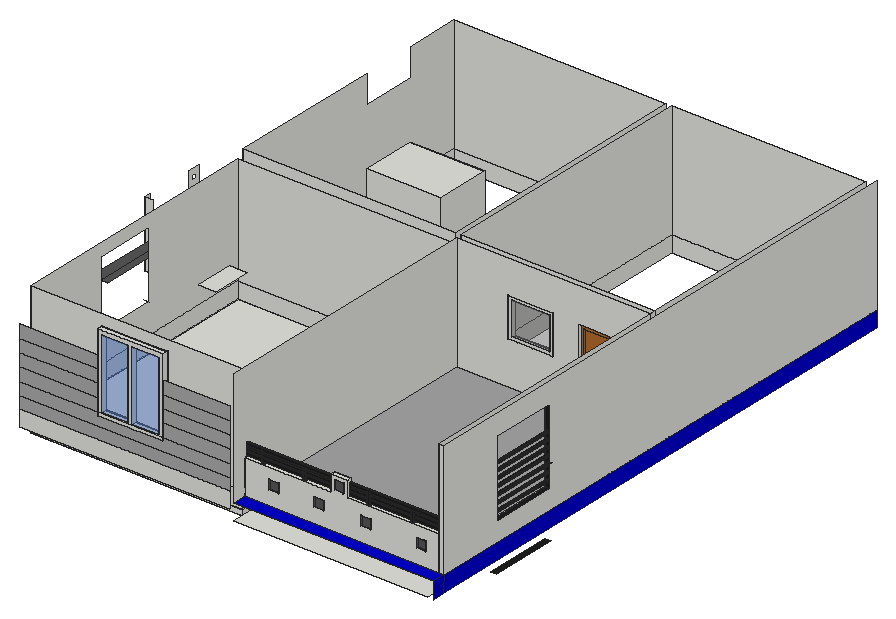
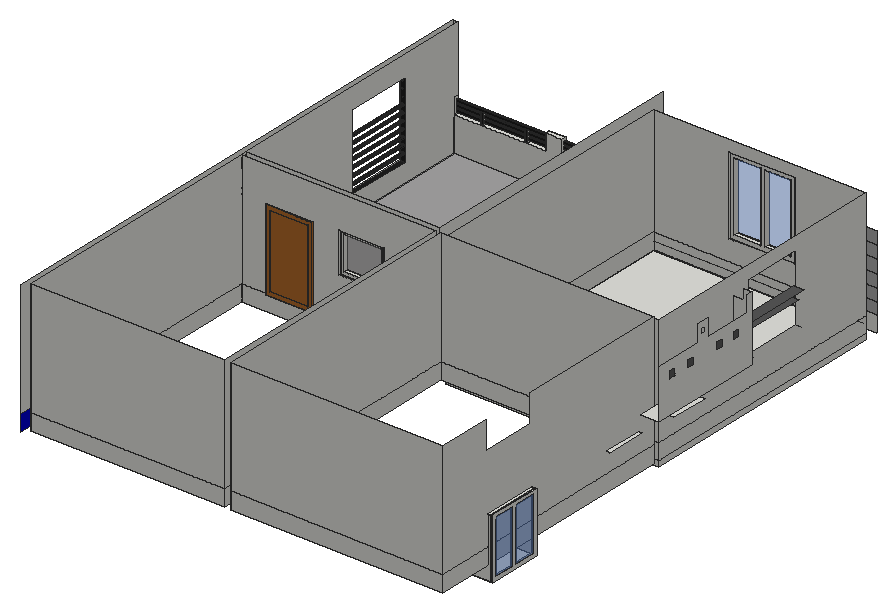
# SketchUp Ruby script. Lengths in inches.
U = 1.inch
M = Sketchup.active_model
def pt(a) = Geom::Point3d.new(a.map { |v| v * U })
def face(e, loops, mat)
  f = e.add_face(loops[0].map { |a| pt(a) })
  loops[1..].each { |l| e.add_face(l.map { |a| pt(a) }).erase! }
  f.material = f.back_material = mat if mat
  f
end
# faces: each face lists its corners as indices into pts; further lists are holes
def faces(e, pts, list, mat = nil) = list.each { |f| face(e, (f[0].is_a?(Array) ? f : [f]).map { |l| l.map { |i| pts[i] } }, mat) }
# xy, xz, yz: faces in a plane at the given z, y or x. An outline is a flat list of corners, or four numbers for a rectangle; further outlines are holes
def ring(l) = l.size == 4 ? [[l[0], l[1]], [l[2], l[1]], [l[2], l[3]], [l[0], l[3]]] : l.each_slice(2).to_a
def flat(e, list, mat, &to3) = list.each { |f| face(e, (f[0].is_a?(Array) ? f : [f]).map { |l| ring(l).map { |u, v| to3.(u, v) } }, mat) }
def xy(e, z, list, mat = nil) = flat(e, list, mat) { |x, y| [x, y, z] }
def xz(e, y, list, mat = nil) = flat(e, list, mat) { |x, z| [x, y, z] }
def yz(e, x, list, mat = nil) = flat(e, list, mat) { |y, z| [x, y, z] }
def lines(e, pts, list) = list.each { |a, b| e.add_line(pt(pts[a]), pt(pts[b])) }
# prism: a flat outline (further loops are holes) pulled along v
def prism(e, loops, v, mat = nil)
  f = face(e, loops, mat); d = Geom::Vector3d.new(v.map { |x| x * U })
  f.pushpull(f.normal.samedirection?(d) ? d.length : -d.length)
end
def box(e, o, s, mat = nil) = prism(e, [[o, [o[0] + s[0], o[1], o[2]], [o[0] + s[0], o[1] + s[1], o[2]], [o[0], o[1] + s[1], o[2]]]], [0, 0, s[2]], mat)
def at(x, y, z, deg = 0) = Geom::Transformation.translation(pt([x, y, z])) * Geom::Transformation.rotation(ORIGIN, Z_AXIS, deg.degrees)
def axes(o, x, y, z) = Geom::Transformation.new([*x, 0, *y, 0, *z, 0, *pt(o).to_a, 1])
def part(name) = M.definitions.add(name)
# library, detail: a bought-in or finely detailed component or shape, given as its bounding box
def library(name, o, s) = part(name).tap { |d| box(d.entities, o, s) }
def detail(e, o, s) = box(e.add_group.entities, o, s)
def put(e, d, t, mat = nil) = e.add_instance(d, t).tap { |i| i.material = mat if mat }
def group(e, t, mat = nil) = e.add_group.tap { |g| g.transformation = t; g.material = mat if mat }.entities
root = M.entities
M.materials.add("[Color I06]").color = [0, 0, 204]
M.materials.add("[Color M03]").color = [170, 170, 170]
M.materials.add("[Color M06]").color = [86, 86, 86]
M.materials.add("[Color M08]").color = [30, 30, 30]
M.materials.add("[Stone Vein Gray]").color = [166, 165, 165]
M.materials.add("[Translucent Glass Blue]").color = [100, 149, 237]
M.materials["[Translucent Glass Blue]"].alpha = 0.5
M.materials.add("[Translucent Glass Gray]").color = [128, 128, 128]
M.materials["[Translucent Glass Gray]"].alpha = 0.5
M.materials.add("[Wood Bamboo]").color = [177, 105, 43]
c1 = part("Group\#2")
xy(c1.entities,0,[[0,0,37.8125,5]])
xy(c1.entities,2.57,[[2.57,0,17.37,5],[19.91,0,35.24,5]])
xy(c1.entities,44.8,[[2.57,0,17.37,5],[19.91,0,35.24,5]])
xy(c1.entities,47.375,[[0,0,37.8125,5]])
xz(c1.entities,0,[[[0,0,37.8125,47.375],[19.91,2.57,35.24,44.8],[2.57,2.57,17.37,44.8]]])
xz(c1.entities,0,[[2.57,2.57,17.37,44.8],[19.91,2.57,35.24,44.8]],"[Translucent Glass Blue]")
xz(c1.entities,5,[[[0,0,37.8125,47.375],[19.91,2.57,35.24,44.8],[2.57,2.57,17.37,44.8]]])
yz(c1.entities,0,[[0,0,5,47.375]])
yz(c1.entities,2.57,[[0,2.57,5,44.8]])
yz(c1.entities,17.37,[[0,2.57,5,44.8]])
yz(c1.entities,19.91,[[0,2.57,5,44.8]])
yz(c1.entities,35.24,[[0,2.57,5,44.8]])
yz(c1.entities,37.8125,[[0,0,5,47.375]])
c2 = part("Group\#1")
xy(c2.entities,0,[[0,0,48,1.5625],[0,1.5625,48,7.5625]],"[Wood Bamboo]")
xy(c2.entities,3.79,[[3.79,0,44.21,1.5625],[3.79,1.5625,44.21,7.5625]],"[Wood Bamboo]")
xy(c2.entities,80.21,[[3.79,0,44.21,1.5625]])
xy(c2.entities,80.21,[[3.79,1.5625,44.21,7.5625]],"[Wood Bamboo]")
xy(c2.entities,84,[[0,0,48,7.5625]],"[Wood Bamboo]")
xz(c2.entities,0,[[[0,0,48,84],[3.79,3.79,44.21,80.21]]],"[Wood Bamboo]")
xz(c2.entities,1.5625,[[3.79,3.79,44.21,80.21]],"[Wood Bamboo]")
xz(c2.entities,7.5625,[[[0,0,48,84],[3.79,3.79,44.21,80.21]],[3.79,3.79,44.21,80.21]],"[Wood Bamboo]")
yz(c2.entities,0,[[0,0,7.5625,84]],"[Wood Bamboo]")
yz(c2.entities,3.79,[[0,3.79,1.5625,80.21],[1.5625,3.79,7.5625,80.21]],"[Wood Bamboo]")
yz(c2.entities,44.21,[[0,3.79,1.5625,80.21],[1.5625,3.79,7.5625,80.21]],"[Wood Bamboo]")
yz(c2.entities,48,[[0,0,7.5625,84]],"[Wood Bamboo]")
c3 = part("Group\#4")
xy(c3.entities,0,[[0,0,32.875,4]])
xy(c3.entities,2.47,[[2.47,0,30.4,4]])
xy(c3.entities,30.4,[[2.47,0,30.4,4]])
xy(c3.entities,32.875,[[0,0,32.875,4]])
xz(c3.entities,0,[[[0,0,32.875,32.875],[2.47,2.47,30.4,30.4]]])
xz(c3.entities,0,[[2.47,2.47,30.4,30.4]],"[Translucent Glass Gray]")
xz(c3.entities,4,[[[0,0,32.875,32.875],[2.47,2.47,30.4,30.4]]])
yz(c3.entities,0,[[0,0,4,32.875]])
yz(c3.entities,2.47,[[0,2.47,4,30.4]])
yz(c3.entities,30.4,[[0,2.47,4,30.4]])
yz(c3.entities,32.875,[[0,0,4,32.875]])
xy(root,252.44,[[77.4375,498.5625,161.6875,555.5]])
xy(root,253.54,[[512.75,125.55,518.75,195.62]],"[Color M08]")
xy(root,260,[[83.4375,62.875,304.75,332.8125]])
xy(root,266,[[310.75,42.6875,512.75,332.8125],[83.4375,62.875,304.75,332.8125]])
xy(root,283,[[310.75,56.875,512.75,62.01],[486.18,332.8125,512.75,338.8125]])
xy(root,283,[[310.75,42.6875,518.75,56.875]],"[Color I06]")
xy(root,283,[[310.75,62.01,512.75,62.01,512.75,332.8125,486.18,332.8125,486.18,338.8125,438.18,338.8125,438.18,332.8125,310.75,332.8125]],"[Stone Vein Gray]")
xy(root,297.98,[[336,56.875,346.32,58.125],[382.57,56.875,392.88,58.3125],[432.32,56.875,442.63,58.25],[489.75,56.875,500.07,58.3125]],"[Color M06]")
xy(root,302.3,[[512.75,125.25,518.75,194.63]],"[Color M08]")
xy(root,302.91,[[77.4375,279.8125,103.125,319.875]])
xy(root,304.56,[[157.85,56.875,226.03,62.875]])
xy(root,308.29,[[336,56.875,346.32,58.125],[382.57,56.875,392.88,58.3125],[432.32,56.875,442.63,58.25],[489.75,56.875,500.07,58.3125]],"[Color M06]")
xy(root,314.88,[[77.4375,498.5625,161.6875,555.5]])
xy(root,319,[[[310.75,56.875,400.84,62.01],[327.84,58.375,330.34,60.875],[370.84,58.375,373.34,60.875]],[[417.89,56.875,512.75,62.01],[436.875,57.96,439.9375,61.02],[483.125,57.96,486.1875,61.02]]])
xy(root,321.07,[[310.75,58.25,512.75,60.56]],"[Color M08]")
xy(root,321.65,[[404.4,56.875,414.08,57.625]],"[Color M06]")
xy(root,323.27,[[59.3125,385.09,62.5,426.22]])
xy(root,323.94,[[310.75,58.25,512.75,60.56]],"[Color M08]")
xy(root,323.97,[[59.3125,241.6875,77.4375,362.77]])
xy(root,325.94,[[310.5625,58.25,512.75,60.56]],"[Color M08]")
xy(root,327.22,[[364.5,332.8125,411.32,338.8125]])
xy(root,328.82,[[310.5625,58.25,512.75,60.56]],"[Color M08]")
xy(root,330.3125,[[370.84,58.375,373.34,60.875]],"[Color M08]")
xy(root,330.44,[[310.75,58.25,512.75,60.56]],"[Color M08]")
xy(root,330.5625,[[483.125,57.96,486.1875,61.02]])
xy(root,331,[[436.875,57.96,439.9375,61.02]])
xy(root,331.625,[[327.84,58.375,330.34,60.875]])
xy(root,332.22,[[404.4,56.875,414.08,57.625]],"[Color M06]")
xy(root,333.32,[[310.75,58.25,512.75,60.56]],"[Color M08]")
xy(root,335.25,[[400.84,56.875,417.89,62.01]])
xy(root,350.58,[[67.1875,170.55,77.4375,235.42]],"[Color M06]")
xy(root,356.84,[[67.1875,164.28,77.4375,241.6875]],"[Color M06]")
xz(root,56.875,[[77.4375,266,295.25,283],[512.75,266,518.75,283],[[310.75,283,512.75,283,512.75,319,417.89,319,417.89,335.25,400.84,335.25,400.84,319,310.75,319],[336,297.98,346.32,308.29],[382.57,297.98,392.88,308.29],[432.32,297.98,442.63,308.29],[489.75,297.98,500.07,308.29],[404.4,321.65,414.08,332.22]],[512.75,283,518.75,403]])
xz(root,56.875,[[77.4375,283,295.25,295.0625],[77.4375,295.0625,295.25,295.0625,295.25,308.13,226.03,308.13,226.03,304.56,157.85,304.56,157.85,308.13,77.4375,308.13],[77.4375,308.13,157.85,321.51],[226.03,308.13,295.25,321.51],[77.4375,321.51,157.85,334.88],
  [226.03,321.51,295.25,334.88],[77.4375,334.88,157.85,348.26],[226.03,334.88,295.25,348.26],[77.4375,348.26,157.85,361.63],[226.03,348.26,295.25,361.63]],"[Color M03]")
xz(root,57.625,[[404.4,321.65,414.08,332.22]],"[Color M06]")
xz(root,57.96,[[436.875,319,439.9375,331],[483.125,319,486.1875,330.5625]],"[Color M08]")
xz(root,58.125,[[336,297.98,346.32,308.29]],"[Color M06]")
xz(root,58.25,[[432.32,297.98,442.63,308.29]],"[Color M06]")
xz(root,58.25,[[310.75,321.07,512.75,323.94],[310.5625,325.94,512.75,328.82],[310.75,330.44,512.75,333.32]],"[Color M08]")
xz(root,58.3125,[[382.57,297.98,392.88,308.29],[489.75,297.98,500.07,308.29]],"[Color M06]")
xz(root,58.375,[[327.84,319,330.34,331.625],[370.84,319,373.34,330.3125]],"[Color M08]")
xz(root,60.56,[[310.75,321.07,512.75,323.94],[310.5625,325.94,512.75,328.82],[310.75,330.44,512.75,333.32]],"[Color M08]")
xz(root,60.875,[[327.84,319,330.34,331.625],[370.84,319,373.34,330.3125]],"[Color M08]")
xz(root,61.02,[[436.875,319,439.9375,331],[483.125,319,486.1875,330.5625]],"[Color M08]")
xz(root,62.01,[[310.75,283,310.75,319,400.84,319,400.84,335.25,417.89,335.25,417.89,319,512.75,319,512.75,283]])
xz(root,62.875,[[83.4375,260,304.75,266],[83.4375,266,304.75,283],[[83.4375,283,304.75,397],[157.85,304.56,226.03,385.87]]])
xz(root,125.25,[[516.02,308.35,516.36,308.4,516.67,308.53,516.95,308.74,517.15,309.01,517.29,309.33,517.33,309.67,517.29,310.01,517.15,310.32,516.95,310.59,516.67,310.8,516.36,310.93,516.02,310.98,515.68,310.93,515.36,310.8,515.09,310.59,514.88,310.32,514.75,310.01,514.71,309.67,514.75,309.33,514.88,309.01,515.09,308.74,515.36,308.53,515.68,308.4],[516.02,315.92,516.36,315.96,516.67,316.09,516.95,316.3,517.15,316.57,517.29,316.89,517.33,317.23,517.29,317.57,517.15,317.88,516.95,318.16,516.67,318.36,516.36,318.5,516.02,318.54,515.68,318.5,515.36,318.36,515.09,318.16,514.88,317.88,514.75,317.57,514.71,317.23,514.75,316.89,514.88,316.57,515.09,316.3,515.36,316.09,515.68,315.96],[516.02,323.48,516.36,323.52,516.67,323.65,516.95,323.86,517.15,324.13,517.29,324.45,517.33,324.79,517.29,325.13,517.15,325.45,516.95,325.72,516.67,325.93,516.36,326.06,516.02,326.1,515.68,326.06,515.36,325.93,515.09,325.72,514.88,325.45,514.75,325.13,514.71,324.79,514.75,324.45,514.88,324.13,515.09,323.86,515.36,323.65,515.68,323.52],[516.02,331.04,516.36,331.09,516.67,331.22,516.95,331.43,517.15,331.7,517.29,332.01,517.33,332.35,517.29,332.69,517.15,333.01,516.95,333.28,516.67,333.49,516.36,333.62,516.02,333.67,515.68,333.62,515.36,333.49,515.09,333.28,514.88,333.01,514.75,332.69,514.71,332.35,514.75,332.01,514.88,331.7,515.09,331.43,515.36,331.22,515.68,331.09],[516.02,338.6,516.36,338.65,516.67,338.78,516.95,338.99,517.15,339.26,517.29,339.58,517.33,339.92,517.29,340.26,517.15,340.57,516.95,340.84,516.67,341.05,516.36,341.18,516.02,341.23,515.68,341.18,515.36,341.05,515.09,340.84,514.88,340.57,514.75,340.26,514.71,339.92,514.75,339.58,514.88,339.26,515.09,338.99,515.36,338.78,515.68,338.65],
  [516.02,346.17,516.36,346.21,516.67,346.34,516.95,346.55,517.15,346.82,517.29,347.14,517.33,347.48,517.29,347.82,517.15,348.13,516.95,348.41,516.67,348.61,516.36,348.75,516.02,348.79,515.68,348.75,515.36,348.61,515.09,348.41,514.88,348.13,514.75,347.82,514.71,347.48,514.75,347.14,514.88,346.82,515.09,346.55,515.36,346.34,515.68,346.21],[516.02,353.73,516.36,353.77,516.67,353.9,516.95,354.11,517.15,354.38,517.29,354.7,517.33,355.04,517.29,355.38,517.15,355.7,516.95,355.97,516.67,356.18,516.36,356.31,516.02,356.35,515.68,356.31,515.36,356.18,515.09,355.97,514.88,355.7,514.75,355.38,514.71,355.04,514.75,354.7,514.88,354.38,515.09,354.11,515.36,353.9,515.68,353.77]])
xz(root,125.25,[[[512.75,302.3,518.75,382.24],[516.02,376.42,516.36,376.46,516.67,376.59,516.95,376.8,517.15,377.07,517.29,377.39,517.33,377.73,517.29,378.07,517.15,378.38,516.95,378.66,516.67,378.86,516.36,379,516.02,379.04,515.68,379,515.36,378.86,515.09,378.66,514.88,378.38,514.75,378.07,514.71,377.73,514.75,377.39,514.88,377.07,515.09,376.8,515.36,376.59,515.68,376.46],[516.02,368.85,516.36,368.9,516.67,369.03,516.95,369.24,517.15,369.51,517.29,369.83,517.33,370.17,517.29,370.51,517.15,370.82,516.95,371.09,516.67,371.3,516.36,371.43,516.02,371.48,515.68,371.43,515.36,371.3,515.09,371.09,514.88,370.82,514.75,370.51,514.71,370.17,514.75,369.83,514.88,369.51,515.09,369.24,515.36,369.03,515.68,368.9],[516.02,361.29,516.36,361.34,516.67,361.47,516.95,361.68,517.15,361.95,517.29,362.26,517.33,362.6,517.29,362.94,517.15,363.26,516.95,363.53,516.67,363.74,516.36,363.87,516.02,363.92,515.68,363.87,515.36,363.74,515.09,363.53,514.88,363.26,514.75,362.94,514.71,362.6,514.75,362.26,514.88,361.95,515.09,361.68,515.36,361.47,515.68,361.34],[516.02,353.73,516.36,353.77,516.67,353.9,516.95,354.11,517.15,354.38,517.29,354.7,517.33,355.04,517.29,355.38,517.15,355.7,516.95,355.97,516.67,356.18,516.36,356.31,516.02,356.35,515.68,356.31,515.36,356.18,515.09,355.97,514.88,355.7,514.75,355.38,514.71,355.04,514.75,354.7,514.88,354.38,515.09,354.11,515.36,353.9,515.68,353.77],[516.02,346.17,516.36,346.21,516.67,346.34,516.95,346.55,517.15,346.82,517.29,347.14,517.33,347.48,517.29,347.82,517.15,348.13,516.95,348.41,516.67,348.61,516.36,348.75,516.02,348.79,515.68,348.75,515.36,348.61,515.09,348.41,514.88,348.13,514.75,347.82,514.71,347.48,514.75,347.14,514.88,346.82,515.09,346.55,515.36,346.34,515.68,346.21],[516.02,338.6,516.36,338.65,516.67,338.78,516.95,338.99,517.15,339.26,517.29,339.58,517.33,339.92,517.29,340.26,517.15,340.57,516.95,340.84,516.67,341.05,516.36,341.18,516.02,341.23,515.68,341.18,515.36,341.05,515.09,340.84,514.88,340.57,514.75,340.26,514.71,339.92,514.75,339.58,514.88,339.26,515.09,338.99,515.36,338.78,515.68,338.65],[516.02,331.04,516.36,331.09,516.67,331.22,516.95,331.43,517.15,331.7,517.29,332.01,517.33,332.35,517.29,332.69,517.15,333.01,516.95,333.28,516.67,333.49,516.36,333.62,516.02,333.67,515.68,333.62,515.36,333.49,515.09,333.28,514.88,333.01,514.75,332.69,514.71,332.35,514.75,332.01,514.88,331.7,515.09,331.43,515.36,331.22,515.68,331.09],[516.02,323.48,516.36,323.52,516.67,323.65,516.95,323.86,517.15,324.13,517.29,324.45,517.33,324.79,517.29,325.13,517.15,325.45,516.95,325.72,516.67,325.93,516.36,326.06,516.02,326.1,515.68,326.06,515.36,325.93,515.09,325.72,514.88,325.45,514.75,325.13,514.71,324.79,514.75,324.45,514.88,324.13,515.09,323.86,515.36,323.65,515.68,323.52],[516.02,315.92,516.36,315.96,516.67,316.09,516.95,316.3,517.15,316.57,517.29,316.89,517.33,317.23,517.29,317.57,517.15,317.88,516.95,318.16,516.67,318.36,516.36,318.5,516.02,318.54,515.68,318.5,515.36,318.36,515.09,318.16,514.88,317.88,514.75,317.57,514.71,317.23,514.75,316.89,514.88,316.57,515.09,316.3,515.36,316.09,515.68,315.96],[516.02,308.35,516.36,308.4,516.67,308.53,516.95,308.74,517.15,309.01,517.29,309.33,517.33,309.67,517.29,310.01,517.15,310.32,516.95,310.59,516.67,310.8,516.36,310.93,516.02,310.98,515.68,310.93,515.36,310.8,515.09,310.59,514.88,310.32,514.75,310.01,514.71,309.67,514.75,309.33,514.88,309.01,515.09,308.74,515.36,308.53,515.68,308.4]]],"[Color M08]")
xz(root,194.63,[[[512.75,302.3,518.75,382.24],[516.02,353.73,515.68,353.77,515.36,353.9,515.09,354.11,514.88,354.38,514.75,354.7,514.71,355.04,514.75,355.38,514.88,355.7,515.09,355.97,515.36,356.18,515.68,356.31,516.02,356.35,516.36,356.31,516.67,356.18,516.95,355.97,517.15,355.7,517.29,355.38,517.33,355.04,517.29,354.7,517.15,354.38,516.95,354.11,516.67,353.9,516.36,353.77],[516.02,346.17,515.68,346.21,515.36,346.34,515.09,346.55,514.88,346.82,514.75,347.14,514.71,347.48,514.75,347.82,514.88,348.13,515.09,348.41,515.36,348.61,515.68,348.75,516.02,348.79,516.36,348.75,516.67,348.61,516.95,348.41,517.15,348.13,517.29,347.82,517.33,347.48,517.29,347.14,517.15,346.82,516.95,346.55,516.67,346.34,516.36,346.21]]],"[Color M08]")
xz(root,194.82,[[516.02,315.92,515.68,315.96,515.36,316.09,515.09,316.3,514.88,316.57,514.75,316.89,514.71,317.23,514.75,317.57,514.88,317.88,515.09,318.16,515.36,318.36,515.68,318.5,516.02,318.54,516.36,318.5,516.67,318.36,516.95,318.16,517.15,317.88,517.29,317.57,517.33,317.23,517.29,316.89,517.15,316.57,516.95,316.3,516.67,316.09,516.36,315.96]])
xz(root,194.88,[[516.02,308.35,515.68,308.4,515.36,308.53,515.09,308.74,514.88,309.01,514.75,309.33,514.71,309.67,514.75,310.01,514.88,310.32,515.09,310.59,515.36,310.8,515.68,310.93,516.02,310.98,516.36,310.93,516.67,310.8,516.95,310.59,517.15,310.32,517.29,310.01,517.33,309.67,517.29,309.33,517.15,309.01,516.95,308.74,516.67,308.53,516.36,308.4]])
xz(root,194.94,[[516.02,331.04,515.68,331.09,515.36,331.22,515.09,331.43,514.88,331.7,514.75,332.01,514.71,332.35,514.75,332.69,514.88,333.01,515.09,333.28,515.36,333.49,515.68,333.62,516.02,333.67,516.36,333.62,516.67,333.49,516.95,333.28,517.15,333.01,517.29,332.69,517.33,332.35,517.29,332.01,517.15,331.7,516.95,331.43,516.67,331.22,516.36,331.09]])
xz(root,195.44,[[516.02,338.6,515.68,338.65,515.36,338.78,515.09,338.99,514.88,339.26,514.75,339.58,514.71,339.92,514.75,340.26,514.88,340.57,515.09,340.84,515.36,341.05,515.68,341.18,516.02,341.23,516.36,341.18,516.67,341.05,516.95,340.84,517.15,340.57,517.29,340.26,517.33,339.92,517.29,339.58,517.15,339.26,516.95,338.99,516.67,338.78,516.36,338.65]])
xz(root,198.94,[[516.02,323.48,515.68,323.52,515.36,323.65,515.09,323.86,514.88,324.13,514.75,324.45,514.71,324.79,514.75,325.13,514.88,325.45,515.09,325.72,515.36,325.93,515.68,326.06,516.02,326.1,516.36,326.06,516.67,325.93,516.95,325.72,517.15,325.45,517.29,325.13,517.33,324.79,517.29,324.45,517.15,324.13,516.95,323.86,516.67,323.65,516.36,323.52]])
xz(root,241.6875,[[59.3125,323.97,67.1875,323.97,67.1875,356.84,77.4375,356.84,77.4375,382.11,67.1875,382.11,67.1875,392.36,59.3125,392.36],[67.1875,323.97,77.4375,356.84]])
xz(root,332.8125,[[83.4375,260,95.93,266],[95.93,260,120.12,266],[120.12,260,304.75,266],[83.4375,266,304.75,283],[83.4375,283,304.75,397],
  [[310.75,283,438.18,283,438.18,367,486.18,367,486.18,283,512.75,283,512.75,403,310.75,403],[364.5,327.22,411.32,368.47]]])
xz(root,338.8125,[[83.4375,266,304.75,283],[310.75,266,512.75,283],[83.4375,283,304.75,403],[[310.75,283,310.75,403,512.75,403,512.75,283,486.18,283,486.18,367,438.18,367,438.18,283],[364.5,327.22,411.32,368.47]]])
xz(root,498.5625,[[77.4375,252.44,161.6875,314.88]])
xz(root,555.5,[[77.4375,252.44,161.6875,314.88]])
xz(root,613.125,[[83.4375,266,304.75,283],[310.75,266,512.75,283],[83.4375,283,304.75,403],[310.75,283,512.75,403]])
yz(root,59.3125,[[[241.6875,323.97,241.6875,392.36,248.07,392.36,248.07,375.04,298.6,375.04,298.6,392.36,311.55,392.36,311.55,375.04,362.77,375.04,362.77,323.97],[341.21,356.93,349.77,365.49],[317.15,356.93,325.71,365.49],[279.4,356.93,287.96,365.49],[258.02,356.93,266.59,365.49],[302.34,381.29,307.53,386.48]]])
yz(root,59.3125,[[258.02,356.93,266.59,365.49],[279.4,356.93,287.96,365.49],[317.15,356.93,325.71,365.49],[341.21,356.93,349.77,365.49]],"[Color M06]")
yz(root,83.4375,[[62.875,260,332.8125,266],[62.875,266,332.8125,283],[338.8125,266,613.125,283],[[62.875,283,332.8125,397],[153.86,314.04,217.18,383.85]],[338.8125,283,613.125,283,613.125,403,556.96,403,556.96,373.64,500.02,373.64,500.02,403,338.8125,403]])
yz(root,157.85,[[56.875,304.56,62.875,385.87]])
yz(root,161.6875,[[498.5625,252.44,555.5,314.88]])
yz(root,226.03,[[56.875,304.56,62.875,385.87]])
yz(root,304.75,[[62.875,260,332.8125,266],[62.875,266,332.8125,283],[338.8125,266,613.125,283],[62.875,283,332.8125,397],[338.8125,283,613.125,403]])
yz(root,310.5625,[[58.25,325.94,60.56,328.82]])
yz(root,310.75,[[338.8125,266,613.125,283],[[42.6875,283,56.875,283,56.875,319,62.01,319,62.01,283,332.8125,283,332.8125,403,42.6875,403],[58.25,330.44,60.56,333.32],[58.25,321.07,60.56,323.94]],[56.875,283,62.01,319],[338.8125,283,613.125,403]])
yz(root,327.84,[[58.375,319,60.875,331.625]],"[Color M08]")
yz(root,330.34,[[58.375,319,60.875,331.625]],"[Color M08]")
yz(root,336,[[56.875,297.98,58.125,308.29]],"[Color M06]")
yz(root,346.32,[[56.875,297.98,58.125,308.29]],"[Color M06]")
yz(root,364.5,[[332.8125,327.22,338.8125,368.47]])
yz(root,370.84,[[58.375,319,60.875,330.3125]])
yz(root,373.34,[[58.375,319,60.875,330.3125]],"[Color M08]")
yz(root,382.57,[[56.875,297.98,58.3125,308.29]],"[Color M06]")
yz(root,392.88,[[56.875,297.98,58.3125,308.29]],"[Color M06]")
yz(root,400.84,[[56.875,319,62.01,335.25]])
yz(root,404.4,[[56.875,321.65,57.625,332.22]],"[Color M06]")
yz(root,411.32,[[332.8125,327.22,338.8125,368.47]])
yz(root,414.08,[[56.875,321.65,57.625,332.22]],"[Color M06]")
yz(root,417.89,[[56.875,319,62.01,335.25]])
yz(root,432.32,[[56.875,297.98,58.25,308.29]],"[Color M06]")
yz(root,436.875,[[57.96,319,61.02,331]])
yz(root,438.18,[[332.8125,283,338.8125,367]])
yz(root,439.9375,[[57.96,319,61.02,331]],"[Color M08]")
yz(root,442.63,[[56.875,297.98,58.25,308.29]],"[Color M06]")
yz(root,483.125,[[57.96,319,61.02,330.5625]])
yz(root,486.18,[[332.8125,283,338.8125,367]])
yz(root,486.1875,[[57.96,319,61.02,330.5625]],"[Color M08]")
yz(root,489.75,[[56.875,297.98,58.3125,308.29]],"[Color M06]")
yz(root,500.07,[[56.875,297.98,58.3125,308.29]],"[Color M06]")
yz(root,512.75,[[56.875,266,338.8125,283],[338.8125,266,613.125,283],[56.875,283,62.01,319],[[62.01,283,62.01,335.25,56.875,335.25,56.875,403,332.8125,403,332.8125,283],[125.25,302.3,194.63,382.24]],[332.8125,283,338.8125,403],
  [338.8125,283,613.125,403],[[56.875,319,62.01,335.25],[58.25,330.44,60.56,333.32],[58.25,325.94,60.56,328.82],[58.25,321.07,60.56,323.94]]])
yz(root,518.75,[[[56.875,283,619.125,403],[125.25,302.3,194.63,382.24]]])
yz(root,518.75,[[42.6875,266,56.875,283],[56.875,266,619.125,283]],"[Color I06]")
p = [[515.68,125.25,308.4],[515.36,125.25,308.53],[515.36,194.88,308.53],[515.68,194.88,308.4],[516.02,125.25,308.35],[516.02,194.88,308.35],
  [516.36,125.25,308.4],[516.36,194.88,308.4],[516.67,125.25,308.53],[516.67,194.88,308.53],[515.09,125.25,308.74],[515.09,194.88,308.74],
  [516.95,125.25,308.74],[516.95,194.88,308.74],[514.88,125.25,309.01],[514.88,194.88,309.01],[517.15,125.25,309.01],[517.15,194.88,309.01],
  [514.75,125.25,309.33],[514.75,194.88,309.33],[517.29,125.25,309.33],[517.29,194.88,309.33],[514.71,125.25,309.67],[514.71,194.88,309.67],
  [517.33,125.25,309.67],[517.33,194.88,309.67],[514.75,125.25,310.01],[514.75,194.88,310.01],[517.29,125.25,310.01],[517.29,194.88,310.01],
  [514.88,125.25,310.32],[514.88,194.88,310.32],[517.15,125.25,310.32],[517.15,194.88,310.32],[515.09,125.25,310.59],[515.09,194.88,310.59],
  [516.95,125.25,310.59],[516.95,194.88,310.59],[515.36,125.25,310.8],[515.36,194.88,310.8],[516.67,125.25,310.8],[516.67,194.88,310.8],
  [515.68,125.25,310.93],[515.68,194.88,310.93],[516.36,125.25,310.93],[516.36,194.88,310.93],[516.02,125.25,310.98],[516.02,194.88,310.98],
  [516.02,125.25,315.92],[515.68,125.25,315.96],[515.68,194.82,315.96],[516.02,194.82,315.92],[516.36,125.25,315.96],[516.36,194.82,315.96],
  [515.36,125.25,316.09],[515.36,194.82,316.09],[516.67,125.25,316.09],[516.67,194.82,316.09],[515.09,125.25,316.3],[515.09,194.82,316.3],
  [516.95,125.25,316.3],[516.95,194.82,316.3],[514.88,125.25,316.57],[514.88,194.82,316.57],[517.15,125.25,316.57],[517.15,194.82,316.57],
  [514.75,125.25,316.89],[514.75,194.82,316.89],[517.29,125.25,316.89],[517.29,194.82,316.89],[514.71,125.25,317.23],[514.71,194.82,317.23],
  [517.33,125.25,317.23],[517.33,194.82,317.23],[514.75,125.25,317.57],[514.75,194.82,317.57],[517.29,125.25,317.57],[517.29,194.82,317.57],
  [514.88,125.25,317.88],[514.88,194.82,317.88],[517.15,125.25,317.88],[517.15,194.82,317.88],[515.09,125.25,318.16],[515.09,194.82,318.16],
  [516.95,125.25,318.16],[516.95,194.82,318.16],[515.36,125.25,318.36],[515.36,194.82,318.36],[516.67,125.25,318.36],[516.67,194.82,318.36],
  [515.68,125.25,318.5],[515.68,194.82,318.5],[516.36,125.25,318.5],[516.36,194.82,318.5],[516.02,125.25,318.54],[516.02,194.82,318.54],
  [515.68,125.25,323.52],[515.36,125.25,323.65],[515.36,198.94,323.65],[515.68,198.94,323.52],[516.02,125.25,323.48],[516.02,198.94,323.48],
  [516.36,125.25,323.52],[516.36,198.94,323.52],[516.67,125.25,323.65],[516.67,198.94,323.65],[515.09,125.25,323.86],[515.09,198.94,323.86],
  [516.95,125.25,323.86],[516.95,198.94,323.86],[514.88,125.25,324.13],[514.88,198.94,324.13],[517.15,125.25,324.13],[517.15,198.94,324.13],
  [514.75,125.25,324.45],[514.75,198.94,324.45],[517.29,125.25,324.45],[517.29,198.94,324.45],[514.71,125.25,324.79],[514.71,198.94,324.79],
  [517.33,125.25,324.79],[517.33,198.94,324.79],[514.75,125.25,325.13],[514.75,198.94,325.13],[517.29,125.25,325.13],[517.29,198.94,325.13],
  [514.88,125.25,325.45],[514.88,198.94,325.45],[517.15,125.25,325.45],[517.15,198.94,325.45],[515.09,125.25,325.72],[515.09,198.94,325.72],
  [516.95,125.25,325.72],[516.95,198.94,325.72],[515.36,125.25,325.93],[515.36,198.94,325.93],[516.67,125.25,325.93],[516.67,198.94,325.93],
  [515.68,125.25,326.06],[515.68,198.94,326.06],[516.36,125.25,326.06],[516.36,198.94,326.06],[516.02,125.25,326.1],[516.02,198.94,326.1],
  [516.02,125.25,331.04],[515.68,125.25,331.09],[515.68,194.94,331.09],[516.02,194.94,331.04],[516.36,125.25,331.09],[516.36,194.94,331.09],
  [515.36,125.25,331.22],[515.36,194.94,331.22],[516.67,125.25,331.22],[516.67,194.94,331.22],[515.09,125.25,331.43],[515.09,194.94,331.43],
  [516.95,125.25,331.43],[516.95,194.94,331.43],[514.88,125.25,331.7],[514.88,194.94,331.7],[517.15,125.25,331.7],[517.15,194.94,331.7],
  [514.75,125.25,332.01],[514.75,194.94,332.01],[517.29,125.25,332.01],[517.29,194.94,332.01],[514.71,125.25,332.35],[514.71,194.94,332.35],
  [517.33,125.25,332.35],[517.33,194.94,332.35],[514.75,125.25,332.69],[514.75,194.94,332.69],[517.29,125.25,332.69],[517.29,194.94,332.69],
  [514.88,125.25,333.01],[514.88,194.94,333.01],[517.15,125.25,333.01],[517.15,194.94,333.01],[515.09,125.25,333.28],[515.09,194.94,333.28],
  [516.95,125.25,333.28],[516.95,194.94,333.28],[515.36,125.25,333.49],[515.36,194.94,333.49],[516.67,125.25,333.49],[516.67,194.94,333.49],
  [515.68,125.25,333.62],[515.68,194.94,333.62],[516.36,125.25,333.62],[516.36,194.94,333.62],[516.02,125.25,333.67],[516.02,194.94,333.67],
  [515.68,125.25,338.65],[515.36,125.25,338.78],[515.36,195.44,338.78],[515.68,195.44,338.65],[516.02,125.25,338.6],[516.02,195.44,338.6],
  [516.36,125.25,338.65],[516.36,195.44,338.65],[516.67,125.25,338.78],[516.67,195.44,338.78],[515.09,125.25,338.99],[515.09,195.44,338.99],
  [516.95,125.25,338.99],[516.95,195.44,338.99],[514.88,125.25,339.26],[514.88,195.44,339.26],[517.15,125.25,339.26],[517.15,195.44,339.26],
  [514.75,125.25,339.58],[514.75,195.44,339.58],[517.29,125.25,339.58],[517.29,195.44,339.58],[514.71,125.25,339.92],[514.71,195.44,339.92],
  [517.33,125.25,339.92],[517.33,195.44,339.92],[514.75,125.25,340.26],[514.75,195.44,340.26],[517.29,125.25,340.26],[517.29,195.44,340.26],
  [514.88,125.25,340.57],[514.88,195.44,340.57],[517.15,125.25,340.57],[517.15,195.44,340.57],[515.09,125.25,340.84],[515.09,195.44,340.84],
  [516.95,125.25,340.84],[516.95,195.44,340.84],[515.36,125.25,341.05],[515.36,195.44,341.05],[516.67,125.25,341.05],[516.67,195.44,341.05],
  [515.68,125.25,341.18],[515.68,195.44,341.18],[516.36,125.25,341.18],[516.36,195.44,341.18],[516.02,125.25,341.23],[516.02,195.44,341.23],
  [515.68,125.25,346.21],[515.36,125.25,346.34],[515.36,194.63,346.34],[515.68,194.63,346.21],[516.02,125.25,346.17],[516.02,194.63,346.17],
  [516.36,125.25,346.21],[516.36,194.63,346.21],[516.67,125.25,346.34],[516.67,194.63,346.34],[515.09,125.25,346.55],[515.09,194.63,346.55],
  [516.95,125.25,346.55],[516.95,194.63,346.55],[514.88,125.25,346.82],[514.88,194.63,346.82],[517.15,125.25,346.82],[517.15,194.63,346.82],
  [514.75,125.25,347.14],[514.75,194.63,347.14],[517.29,125.25,347.14],[517.29,194.63,347.14],[514.71,125.25,347.48],[514.71,194.63,347.48],
  [517.33,125.25,347.48],[517.33,194.63,347.48],[514.75,125.25,347.82],[514.75,194.63,347.82],[517.29,125.25,347.82],[517.29,194.63,347.82],
  [514.88,125.25,348.13],[514.88,194.63,348.13],[517.15,125.25,348.13],[517.15,194.63,348.13],[515.09,125.25,348.41],[515.09,194.63,348.41],
  [516.95,125.25,348.41],[516.95,194.63,348.41],[515.36,125.25,348.61],[515.36,194.63,348.61],[516.67,125.25,348.61],[516.67,194.63,348.61],
  [515.68,125.25,348.75],[515.68,194.63,348.75],[516.36,125.25,348.75],[516.36,194.63,348.75],[516.02,125.25,348.79],[516.02,194.63,348.79],
  [516.02,125.25,353.73],[515.68,125.25,353.77],[515.68,194.63,353.77],[516.02,194.63,353.73],[516.36,125.25,353.77],[516.36,194.63,353.77],
  [515.36,125.25,353.9],[515.36,194.63,353.9],[516.67,125.25,353.9],[516.67,194.63,353.9],[515.09,125.25,354.11],[515.09,194.63,354.11],
  [516.95,125.25,354.11],[516.95,194.63,354.11],[514.88,125.25,354.38],[514.88,194.63,354.38],[517.15,125.25,354.38],[517.15,194.63,354.38],
  [514.75,125.25,354.7],[514.75,194.63,354.7],[517.29,125.25,354.7],[517.29,194.63,354.7],[514.71,125.25,355.04],[514.71,194.63,355.04],
  [517.33,125.25,355.04],[517.33,194.63,355.04],[514.75,125.25,355.38],[514.75,194.63,355.38],[517.29,125.25,355.38],[517.29,194.63,355.38],
  [514.88,125.25,355.7],[514.88,194.63,355.7],[517.15,125.25,355.7],[517.15,194.63,355.7],[515.09,125.25,355.97],[515.09,194.63,355.97],
  [516.95,125.25,355.97],[516.95,194.63,355.97],[515.36,125.25,356.18],[515.36,194.63,356.18],[516.67,125.25,356.18],[516.67,194.63,356.18],
  [515.68,125.25,356.31],[515.68,194.63,356.31],[516.36,125.25,356.31],[516.36,194.63,356.31],[516.02,125.25,356.35],[516.02,194.63,356.35],
  [77.4375,153.86,314.04],[83.4375,153.86,314.04],[77.4375,217.18,314.04],[83.4375,217.18,314.04],[157.85,56.875,308.13],[226.03,56.875,308.13],
  [77.4375,74.1875,283],[83.4375,74.1875,283],[295.25,74.1875,283],[516.67,125.25,300.97],[516.95,125.25,301.18],[516.02,125.25,300.79],
  [516.36,125.25,300.84],[517.15,125.25,301.45],[517.29,125.25,301.76],[517.33,125.25,302.1],[517.3,125.25,302.3],[514.71,125.25,302.1],
  [514.75,125.25,301.76],[514.88,125.25,301.45],[515.09,125.25,301.18],[515.36,125.25,300.97],[515.68,125.25,300.84],[514.73,125.25,302.3],
  [516.67,125.25,293.4],[516.95,125.25,293.61],[516.02,125.25,293.23],[516.36,125.25,293.27],[517.15,125.25,293.88],[517.29,125.25,294.2],
  [517.33,125.25,294.54],[517.29,125.25,294.88],[517.15,125.25,295.2],[516.95,125.25,295.47],[516.67,125.25,295.68],[516.36,125.25,295.81],
  [516.02,125.25,295.85],[515.68,125.25,295.81],[515.36,125.25,295.68],[515.09,125.25,295.47],[514.88,125.25,295.2],[514.75,125.25,294.88],
  [514.71,125.25,294.54],[514.75,125.25,294.2],[514.88,125.25,293.88],[515.09,125.25,293.61],[515.36,125.25,293.4],[515.68,125.25,293.27],
  [516.67,125.25,285.84],[516.95,125.25,286.05],[516.02,125.25,285.67],[516.36,125.25,285.71],[517.15,125.25,286.32],[517.29,125.25,286.64],
  [517.33,125.25,286.98],[517.29,125.25,287.32],[517.15,125.25,287.63],[516.95,125.25,287.91],[516.67,125.25,288.11],[516.36,125.25,288.25],
  [516.02,125.25,288.29],[515.68,125.25,288.25],[515.36,125.25,288.11],[515.09,125.25,287.91],[514.88,125.25,287.63],[514.75,125.25,287.32],
  [514.71,125.25,286.98],[514.75,125.25,286.64],[514.88,125.25,286.32],[515.09,125.25,286.05],[515.36,125.25,285.84],[515.68,125.25,285.71]]
faces(root,p,[[0,1,2,3],[4,0,3,5],[6,4,5,7],[8,6,7,9],[1,10,11,2],[12,8,9,13],[10,14,15,11],[16,12,13,17],
  [14,18,19,15],[20,16,17,21],[18,22,23,19],[24,20,21,25],[22,26,27,23],[28,24,25,29],[26,30,31,27],[32,28,29,33],
  [30,34,35,31],[36,32,33,37],[34,38,39,35],[40,36,37,41],[38,42,43,39],[44,40,41,45],[42,46,47,43],[46,44,45,47],
  [48,49,50,51],[52,48,51,53],[49,54,55,50],[56,52,53,57],[54,58,59,55],[60,56,57,61],[58,62,63,59],[64,60,61,65],
  [62,66,67,63],[68,64,65,69],[66,70,71,67],[72,68,69,73],[70,74,75,71],[76,72,73,77],[74,78,79,75],[80,76,77,81],
  [78,82,83,79],[84,80,81,85],[82,86,87,83],[88,84,85,89],[86,90,91,87],[92,88,89,93],[90,94,95,91],[94,92,93,95],
  [96,97,98,99],[100,96,99,101],[102,100,101,103],[104,102,103,105],[97,106,107,98],[108,104,105,109],[106,110,111,107],[112,108,109,113],
  [110,114,115,111],[116,112,113,117],[114,118,119,115],[120,116,117,121],[118,122,123,119],[124,120,121,125],[122,126,127,123],[128,124,125,129],
  [126,130,131,127],[132,128,129,133],[130,134,135,131],[136,132,133,137],[134,138,139,135],[140,136,137,141],[138,142,143,139],[142,140,141,143],
  [144,145,146,147],[148,144,147,149],[145,150,151,146],[152,148,149,153],[150,154,155,151],[156,152,153,157],[154,158,159,155],[160,156,157,161],
  [158,162,163,159],[164,160,161,165],[162,166,167,163],[168,164,165,169],[166,170,171,167],[172,168,169,173],[170,174,175,171],[176,172,173,177],
  [174,178,179,175],[180,176,177,181],[178,182,183,179],[184,180,181,185],[182,186,187,183],[188,184,185,189],[186,190,191,187],[190,188,189,191],
  [192,193,194,195],[196,192,195,197],[198,196,197,199],[200,198,199,201],[193,202,203,194],[204,200,201,205],[202,206,207,203],[208,204,205,209],
  [206,210,211,207],[212,208,209,213],[210,214,215,211],[216,212,213,217],[214,218,219,215],[220,216,217,221],[218,222,223,219],[224,220,221,225],
  [222,226,227,223],[228,224,225,229],[226,230,231,227],[232,228,229,233],[230,234,235,231],[236,232,233,237],[234,238,239,235],[238,236,237,239],
  [240,241,242,243],[244,240,243,245],[246,244,245,247],[248,246,247,249],[241,250,251,242],[252,248,249,253],[250,254,255,251],[256,252,253,257],
  [254,258,259,255],[260,256,257,261],[258,262,263,259],[264,260,261,265],[262,266,267,263],[268,264,265,269],[266,270,271,267],[272,268,269,273],
  [270,274,275,271],[276,272,273,277],[274,278,279,275],[280,276,277,281],[278,282,283,279],[284,280,281,285],[282,286,287,283],[286,284,285,287],
  [288,289,290,291],[292,288,291,293],[289,294,295,290],[296,292,293,297],[294,298,299,295],[300,296,297,301],[298,302,303,299],[304,300,301,305],
  [302,306,307,303],[308,304,305,309],[306,310,311,307],[312,308,309,313],[310,314,315,311],[316,312,313,317],[314,318,319,315],[320,316,317,321],
  [318,322,323,319],[324,320,321,325],[322,326,327,323],[328,324,325,329],[326,330,331,327],[332,328,329,333],[330,334,335,331],[334,332,333,335]],"[Color M08]")
lines(root,p,[[336,337],[338,339],[340,341],[342,343],[343,344],[345,346],[347,348],[348,345],[346,349],[349,350],[350,351],[351,352],
  [353,354],[354,355],[355,356],[356,357],[357,358],[358,347],[359,353],[360,361],[362,363],[363,360],[361,364],[364,365],
  [365,366],[366,367],[367,368],[368,369],[369,370],[370,371],[371,372],[372,373],[373,374],[374,375],[375,376],[376,377],
  [377,378],[378,379],[379,380],[380,381],[381,382],[382,383],[383,362],[384,385],[386,387],[387,384],[385,388],[388,389],
  [389,390],[390,391],[391,392],[392,393],[393,394],[394,395],[395,396],[396,397],[397,398],[398,399],[399,400],[400,401],
  [401,402],[402,403],[403,404],[404,405],[405,406],[406,407],[407,386]])
put(root,c1,axes([77.4375,555.5,252.44],[0,-1.50579,0],[0.41,0,0],[0,0,1.32058]))
put(root,c2,axes([438.17,334.85,283],[1.0001,0,0],[0,0.73,0],[0,0,1]))
put(root,c1,axes([157.85,56.875,304.56],[1.80331,0,0],[0,1,0],[0,0,1.71636]))
put(root,c3,axes([364.63,332.8125,327.22],[1.42,0,0],[0,1,0],[0,0,1.25475]))
